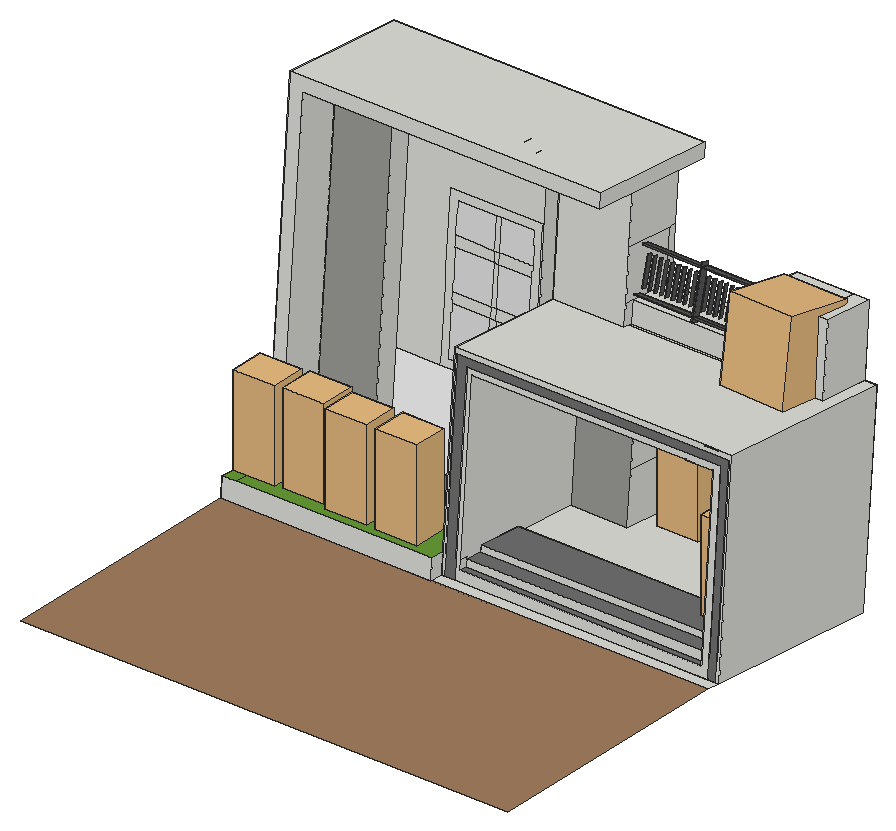
# SketchUp Ruby script. Lengths in inches.
U = 1.inch
M = Sketchup.active_model
def pt(a) = Geom::Point3d.new(a.map { |v| v * U })
def face(e, loops, mat)
  f = e.add_face(loops[0].map { |a| pt(a) })
  loops[1..].each { |l| e.add_face(l.map { |a| pt(a) }).erase! }
  f.material = f.back_material = mat if mat
  f
end
# faces: each face lists its corners as indices into pts; further lists are holes
def faces(e, pts, list, mat = nil) = list.each { |f| face(e, (f[0].is_a?(Array) ? f : [f]).map { |l| l.map { |i| pts[i] } }, mat) }
# xy, xz, yz: faces in a plane at the given z, y or x. An outline is a flat list of corners, or four numbers for a rectangle; further outlines are holes
def ring(l) = l.size == 4 ? [[l[0], l[1]], [l[2], l[1]], [l[2], l[3]], [l[0], l[3]]] : l.each_slice(2).to_a
def flat(e, list, mat, &to3) = list.each { |f| face(e, (f[0].is_a?(Array) ? f : [f]).map { |l| ring(l).map { |u, v| to3.(u, v) } }, mat) }
def xy(e, z, list, mat = nil) = flat(e, list, mat) { |x, y| [x, y, z] }
def xz(e, y, list, mat = nil) = flat(e, list, mat) { |x, z| [x, y, z] }
def yz(e, x, list, mat = nil) = flat(e, list, mat) { |y, z| [x, y, z] }
def lines(e, pts, list) = list.each { |a, b| e.add_line(pt(pts[a]), pt(pts[b])) }
# prism: a flat outline (further loops are holes) pulled along v
def prism(e, loops, v, mat = nil)
  f = face(e, loops, mat); d = Geom::Vector3d.new(v.map { |x| x * U })
  f.pushpull(f.normal.samedirection?(d) ? d.length : -d.length)
end
def box(e, o, s, mat = nil) = prism(e, [[o, [o[0] + s[0], o[1], o[2]], [o[0] + s[0], o[1] + s[1], o[2]], [o[0], o[1] + s[1], o[2]]]], [0, 0, s[2]], mat)
def at(x, y, z, deg = 0) = Geom::Transformation.translation(pt([x, y, z])) * Geom::Transformation.rotation(ORIGIN, Z_AXIS, deg.degrees)
def axes(o, x, y, z) = Geom::Transformation.new([*x, 0, *y, 0, *z, 0, *pt(o).to_a, 1])
def part(name) = M.definitions.add(name)
# library, detail: a bought-in or finely detailed component or shape, given as its bounding box
def library(name, o, s) = part(name).tap { |d| box(d.entities, o, s) }
def detail(e, o, s) = box(e.add_group.entities, o, s)
def put(e, d, t, mat = nil) = e.add_instance(d, t).tap { |i| i.material = mat if mat }
def group(e, t, mat = nil) = e.add_group.tap { |g| g.transformation = t; g.material = mat if mat }.entities
root = M.entities
M.materials.add("M (5)").color = [89, 89, 89]
M.materials.add("M (7)").color = [139, 146, 159]
M.materials.add("[0128_White]").color = [255, 255, 255]
M.materials.add("[Cladding Siding Tan]").color = [162, 126, 95]
M.materials.add("[Color M05]").color = [114, 114, 114]
M.materials.add("[Concrete Block 8x8 Gray]").color = [157, 158, 154]
M.materials.add("[Grass Dark Green]").color = [106, 157, 55]
M.materials.add("[Mirror 02]").color = [229, 229, 229]
c1 = library("Sphere Light",[-0.01,-0.01,-0.01],[0.02,0.02,0.02])
c2 = library("Sphere Light\#2",[-3.2,-3.2,-3.2],[6.4,6.4,6.4])
c3 = library("Sphere Light\#3",[-3.51,-3.51,-3.51],[7.02,7.02,7.02])
c4 = library("Sphere Light\#4",[-3.28,-3.28,-3.28],[6.56,6.56,6.56])
c5 = library("Sphere Light\#6",[-4.5625,-4.5625,-4.5625],[9.125,9.125,9.125])
c6 = library("Sphere Light\#7",[-3.84,-3.84,-3.84],[7.68,7.68,7.68])
c7 = library("Sphere Light\#8",[-4.49,-4.49,-4.49],[8.98,8.98,8.98])
c8 = library("Sphere Light\#9",[-5.16,-5.16,-5.16],[10.32,10.32,10.32])
c9 = library("PINTU+6+YA",[0,-0.6875,0],[35.83,8.07,80.71])
c10 = library("Sphere Light\#10",[-4.25,-4.25,-4.25],[8.5,8.5,8.5])
c11 = library("TS_VASO+GANCHOS-PARA-PENDURAR\#1",[-17.61,-15.74,-70.29],[36.55,50.24,77.96])
c12 = library("Group_2",[-1.28,-0.39,0],[21.22,20.51,48.44])
c13 = library("Sphere Light\#11",[-1.79,-1.79,-1.79],[3.58,3.58,3.58])
c14 = part("Railing post")
box(c14.entities,[0,-0.79,0],[1.18,1.58,46.0625],"M (5)")
c15 = part("Horizontal rails")
box(c15.entities,[0,-0.79,0],[54.52,1.58,1.18],"M (5)")
box(c15.entities,[55.7,-0.79,0],[54.54,1.58,1.18],"M (5)")
xy(c15.entities,38.58,[[55.7,-0.79,58.22,0.79]])
xy(c15.entities,38.58,[[46.34,-0.79,51.99,0.79],[51.99,-0.79,54.52,0.79],[58.22,-0.79,63.67,0.79],[63.67,-0.79,69.12,0.79],[69.12,-0.79,74.57,0.79],
  [74.57,-0.79,80.02,0.79],[80.02,-0.79,85.47,0.79],[85.47,-0.79,90.93,0.79],[90.93,-0.79,96.375,0.79],[96.375,-0.79,101.83,0.79],
  [101.83,-0.79,107.48,0.79],[107.48,-0.79,110.24,0.79]],"M (5)")
xy(c15.entities,38.58,[[0,-0.79,2.73,0.79],[2.73,-0.79,5.45,0.79],[5.45,-0.79,8.18,0.79],[8.18,-0.79,13.63,0.79],[13.63,-0.79,19.08,0.79],
  [19.08,-0.79,24.53,0.79],[24.53,-0.79,29.98,0.79],[29.98,-0.79,35.4375,0.79],[35.4375,-0.79,40.89,0.79],[40.89,-0.79,46.34,0.79]],"M (7)")
xy(c15.entities,39.76,[[0,-0.79,54.52,0.79],[55.7,-0.79,110.24,0.79]],"M (5)")
xz(c15.entities,-0.79,[[0,38.58,54.52,39.76],[55.7,38.58,110.24,39.76]],"M (5)")
xz(c15.entities,0.79,[[0,38.58,54.52,39.76],[55.7,38.58,110.24,39.76]],"M (5)")
yz(c15.entities,0,[[-0.79,38.58,0.79,39.76]],"M (7)")
yz(c15.entities,54.52,[[-0.79,38.58,0.79,39.76]],"M (5)")
yz(c15.entities,55.7,[[-0.79,38.58,0.79,39.76]])
yz(c15.entities,110.24,[[-0.79,38.58,0.79,39.76]],"M (5)")
c16 = part("Railing balusters")
xz(c16.entities,0,[[0,0,0.79,26.38],[5.45,0,6.24,26.38],[10.9,0,11.69,26.38],[16.35,0,17.14,26.38],[21.81,0,22.59,26.38],
  [27.26,0,28.05,26.38],[32.71,0,33.5,26.38],[38.16,0,38.95,26.38],[43.61,0,44.4,26.38],[55.68,0,56.46,26.38],
  [61.13,0,61.91,26.38],[66.58,0,67.37,26.38],[72.03,0,72.82,26.38],[77.48,0,78.27,26.38],[82.93,0,83.72,26.38],
  [88.39,0,89.17,26.38],[93.84,0,94.625,26.38],[99.29,0,100.08,26.38]],"M (5)")
xz(c16.entities,0.79,[[0,0,0.79,26.38],[5.45,0,6.24,26.38],[10.9,0,11.69,26.38],[16.35,0,17.14,26.38],[21.81,0,22.59,26.38],
  [27.26,0,28.05,26.38],[32.71,0,33.5,26.38],[38.16,0,38.95,26.38],[43.61,0,44.4,26.38],[55.68,0,56.46,26.38],
  [61.13,0,61.91,26.38],[66.58,0,67.37,26.38],[72.03,0,72.82,26.38],[77.48,0,78.27,26.38],[82.93,0,83.72,26.38],
  [88.39,0,89.17,26.38],[93.84,0,94.625,26.38],[99.29,0,100.08,26.38]],"M (5)")
yz(c16.entities,0,[[0,0,0.79,26.38]],"M (5)")
yz(c16.entities,0.79,[[0,0,0.79,26.38]],"M (5)")
yz(c16.entities,5.45,[[0,0,0.79,26.38]],"M (5)")
yz(c16.entities,6.24,[[0,0,0.79,26.38]],"M (5)")
yz(c16.entities,10.9,[[0,0,0.79,26.38]],"M (5)")
yz(c16.entities,11.69,[[0,0,0.79,26.38]],"M (5)")
yz(c16.entities,16.35,[[0,0,0.79,26.38]],"M (5)")
yz(c16.entities,17.14,[[0,0,0.79,26.38]],"M (5)")
yz(c16.entities,21.81,[[0,0,0.79,26.38]],"M (5)")
yz(c16.entities,22.59,[[0,0,0.79,26.38]],"M (5)")
yz(c16.entities,27.26,[[0,0,0.79,26.38]],"M (5)")
yz(c16.entities,28.05,[[0,0,0.79,26.38]],"M (5)")
yz(c16.entities,32.71,[[0,0,0.79,26.38]],"M (5)")
yz(c16.entities,33.5,[[0,0,0.79,26.38]],"M (5)")
yz(c16.entities,38.16,[[0,0,0.79,26.38]],"M (5)")
yz(c16.entities,38.95,[[0,0,0.79,26.38]],"M (5)")
yz(c16.entities,43.61,[[0,0,0.79,26.38]],"M (5)")
yz(c16.entities,44.4,[[0,0,0.79,26.38]],"M (5)")
yz(c16.entities,55.68,[[0,0,0.79,26.38]],"M (5)")
yz(c16.entities,56.46,[[0,0,0.79,26.38]],"M (5)")
yz(c16.entities,61.13,[[0,0,0.79,26.38]],"M (5)")
yz(c16.entities,61.91,[[0,0,0.79,26.38]],"M (5)")
yz(c16.entities,66.58,[[0,0,0.79,26.38]],"M (5)")
yz(c16.entities,67.37,[[0,0,0.79,26.38]],"M (5)")
yz(c16.entities,72.03,[[0,0,0.79,26.38]],"M (5)")
yz(c16.entities,72.82,[[0,0,0.79,26.38]],"M (5)")
yz(c16.entities,77.48,[[0,0,0.79,26.38]],"M (5)")
yz(c16.entities,78.27,[[0,0,0.79,26.38]],"M (5)")
yz(c16.entities,82.93,[[0,0,0.79,26.38]],"M (5)")
yz(c16.entities,83.72,[[0,0,0.79,26.38]],"M (5)")
yz(c16.entities,88.39,[[0,0,0.79,26.38]],"M (5)")
yz(c16.entities,89.17,[[0,0,0.79,26.38]],"M (5)")
yz(c16.entities,93.84,[[0,0,0.79,26.38]],"M (5)")
yz(c16.entities,94.625,[[0,0,0.79,26.38]],"M (5)")
yz(c16.entities,99.29,[[0,0,0.79,26.38]],"M (5)")
yz(c16.entities,100.08,[[0,0,0.79,26.38]],"M (5)")
xy(root,21.39,[[0,0,181.29,93.04]],"[Cladding Siding Tan]")
yz(root,0,[[162.59,15.42,98.14,20.95,93.04,21.39,93.66,28.68,114.9,26.86,125.41,149.41,173.73,145.27]])
yz(root,5.0625,[[163.22,22.72,163.32,23.92,130.44,26.74,115,28.07,114.9,26.86],[163.32,23.92,173.3,140.22,140.42,143.04,130.44,26.74],[130.44,26.74,140.42,143.04,124.97,144.37,115,28.07]])
yz(root,26.62,[[138.23,26.08,141.13,59.9,148.2,142.375,140.42,143.04,130.44,26.74]])
yz(root,78.16,[[165.15,15.21,162.59,15.42,163.22,22.72,165.77,22.5],[162.59,15.42,163.22,22.72,98.77,28.25,98.14,20.95],[98.14,20.95,98.77,28.25,93.66,28.68,93.04,21.39],[165.77,22.5,163.22,22.72,163.32,23.92,165.875,23.7],[163.22,22.72,98.77,28.25,98.87,29.45,138.23,26.08,163.32,23.92],
  [165.875,23.7,163.32,23.92,173.3,140.22,175.85,140.01],[163.32,23.92,173.3,140.22,154.24,141.86,149.8125,90.23,143.77,90.75,141.13,59.9,138.23,26.08],[138.23,26.08,98.87,29.45,104.42,94.12,143.77,90.75,141.13,59.9],[149.8125,90.23,154.24,141.86,148.2,142.375,143.77,90.75]])
yz(root,79.13,[[100.82,28.07,106.31,92.02,104.25,92.2,98.77,28.25]])
yz(root,83.04,[[100.82,28.07,98.77,28.25,104.02,89.46,106.07,89.28]])
yz(root,84.88,[[149.77,23.87,154.84,83.05,103.84,87.43,98.77,28.25,101.51,28.01,101.46,27.41,107.76,26.87,107.8125,27.47,107.92,28.67,107.96,29.15,125.35,27.66,125.31,27.18,125.2,25.98],[125.2,25.98,107.8125,27.47,107.92,28.67,125.31,27.18],[125.31,27.18,107.92,28.67,107.96,29.15,125.35,27.66]])
yz(root,104.71,[[153.11,89.94,153.76,97.51,150.46,97.8,149.8125,90.23,152.05,90.04],[172.07,95.94,173.64,114.19,171.08,114.41,169.52,96.16],[169.52,96.16,171.08,114.41,152.03,116.04,150.46,97.8,153.76,97.51],[173.64,114.19,175.85,140.01,173.3,140.22,154.24,141.86,152.03,116.04,171.08,114.41]])
yz(root,105.9375,[[165.77,22.5,167.35,40.95,151.35,42.32,149.77,23.87],[167.35,40.95,169.69,68.23,153.69,69.6,151.35,42.32],[169.69,68.23,170.84,81.57,170.85,81.68,154.84,83.05,153.69,69.6]])
yz(root,115.65,[[173.3,140.22,173.73,145.27,125.41,149.41,124.97,144.37]])
yz(root,150.09,[[172.07,95.94,169.52,96.16,171.08,114.41,173.64,114.19],[169.52,96.16,155.82,97.34,157.38,115.58,171.08,114.41],[155.8,97.18,155.82,97.34,153.76,97.51,153.75,97.35]])
yz(root,164.56,[[170.84,81.57,103.83,87.32,103.84,87.43,170.85,81.68]])
yz(root,171.28,[[171.41,88.27,171.42,88.375,168.87,88.59,168.86,88.48],[153.11,89.94,152.05,90.04,152.69,97.44,153.75,97.35],[155.8,97.18,153.75,97.35,152.69,97.44,154.27,115.85,157.38,115.58],[173.64,114.19,157.38,115.58,154.27,115.85,154.28,115.96,173.64,114.3]])
yz(root,174.57,[[[165.77,22.5,125.2,25.98,125.35,27.66,107.96,29.15,107.8125,27.47,107.76,26.87,101.46,27.41,98.72,27.65,103.83,87.32,170.84,81.57],[161.79,43.81,163.9375,68.91,154.16,69.74,152.01,44.65]],[125.2,25.98,125.35,27.66,107.96,29.15,107.8125,27.47],[161.79,43.81,152.01,44.65,154.16,69.74,163.9375,68.91]])
yz(root,176.84,[[171.41,88.27,168.86,88.48,168.87,88.59,171.42,88.375],[171.42,88.375,173.64,114.3,154.28,115.96,152.05,90.04,168.87,88.59]])
yz(root,177.23,[[100.77,27.47,101.37,34.42,99.3125,34.6,98.72,27.65],[101.37,34.42,106.07,89.28,104.02,89.46,99.3125,34.6]])
yz(root,180.19,[[100.77,27.47,98.72,27.65,104.25,92.2,106.31,92.02]])
yz(root,181.29,[[165.15,15.21,171.42,88.375,104.42,94.12,98.14,20.95]])
p = [[78.16,98.14,20.95],[78.16,162.59,15.42],[78.16,165.15,15.21],[181.29,165.15,15.21],[181.29,98.14,20.95],[180.19,98.14,20.95],
  [177.23,98.14,20.95],[83.04,98.14,20.95],[79.13,98.14,20.95],[78.16,175.85,140.01],[78.16,165.875,23.7],[78.16,165.77,22.5],
  [181.29,171.42,88.375],[176.84,171.42,88.375],[176.84,171.41,88.27],[171.28,171.41,88.27],[171.28,171.42,88.375],[176.84,173.64,114.3],
  [171.28,173.64,114.3],[171.28,173.64,114.19],[150.09,173.64,114.19],[150.09,172.07,95.94],[104.71,172.07,95.94],[104.71,173.64,114.19],
  [104.71,175.85,140.01],[105.9375,169.69,68.23],[105.9375,170.84,81.57],[105.9375,170.85,81.68],[164.56,170.85,81.68],[164.56,170.84,81.57],
  [174.57,170.84,81.57],[174.57,165.77,22.5],[105.9375,165.77,22.5],[105.9375,167.35,40.95],[0,98.14,20.95],[0,162.59,15.42],
  [0,173.73,145.27],[115.65,173.73,145.27],[115.65,173.3,140.22],[104.71,173.3,140.22],[78.16,173.3,140.22],[26.62,173.3,140.22],
  [5.0625,173.3,140.22],[5.0625,163.32,23.92],[5.0625,163.22,22.72],[78.16,163.22,22.72],[0,93.04,21.39],[78.16,93.04,21.39],
  [181.29,93.04,21.39],[180.19,104.25,92.2],[180.19,98.72,27.65],[181.29,104.42,94.12],[176.84,104.42,94.12],[176.84,104.41,94.01],
  [171.28,104.41,94.01],[171.28,104.42,94.12],[78.16,104.42,94.12],[78.16,98.87,29.45],[78.16,98.77,28.25],[79.13,98.77,28.25],
  [79.13,104.25,92.2],[178.75,104.25,92.2],[83.04,98.77,28.25],[83.04,104.02,89.46],[177.23,104.02,89.46],[177.23,99.3125,34.6],
  [177.23,98.72,27.65],[174.57,103.83,87.32],[174.57,98.72,27.65],[174.55,98.44,24.41],[84.86,98.49,25.01],[84.88,98.77,28.25],
  [84.88,103.84,87.43],[164.56,103.84,87.43],[164.56,103.83,87.32],[78.16,93.66,28.68],[5.0625,93.66,28.68],[0,93.66,28.68],
  [84.88,149.77,23.87],[84.88,125.2,25.98],[174.57,125.2,25.98],[105.9375,149.77,23.87],[114.1875,169.69,68.23],[114.1875,167.35,40.95],
  [141.68,169.63,67.53],[156.43,169.63,67.53],[156.43,166.55,31.53],[141.68,166.55,31.53],[134.875,166.79,34.34],[123.6875,166.79,34.34],
  [123.6875,169.63,67.53],[134.875,169.63,67.53],[5.0625,114.9,26.86],[78.16,163.32,23.92],[26.62,163.32,23.92],[26.62,138.23,26.08],
  [26.62,130.44,26.74],[5.0625,130.44,26.74],[78.16,138.23,26.08],[105.9375,151.35,42.32],[105.9375,153.69,69.6],[105.9375,154.84,83.05],
  [84.88,154.84,83.05],[174.55,101.18,24.17],[84.86,101.23,24.77],[174.57,101.46,27.41],[84.88,101.46,27.41],[84.88,101.51,28.01],
  [84.88,125.31,27.18],[84.88,125.35,27.66],[174.57,125.35,27.66],[78.16,141.13,59.9],[77.59,141.13,59.9],[43.28,141.13,59.9],
  [26.62,141.13,59.9],[26.62,140.42,143.04],[5.0625,140.42,143.04],[0,114.9,26.86],[174.57,107.76,26.87],[84.88,107.76,26.87],
  [174.57,107.96,29.15],[84.88,107.96,29.15],[84.88,107.92,28.67],[84.88,107.8125,27.47],[174.57,107.8125,27.47],[0,125.41,149.41],
  [5.0625,115,28.07],[5.0625,124.97,144.37],[115.65,124.97,144.37],[115.65,125.41,149.41],[177.23,100.77,27.47],[180.19,100.77,27.47],
  [180.19,106.31,92.02],[178.75,106.31,92.02],[79.13,106.31,92.02],[79.13,100.82,28.07],[83.04,100.82,28.07],[83.04,106.07,89.28],
  [177.23,106.07,89.28],[177.23,101.37,34.42],[77.59,145.99,116.63],[78.16,143.77,90.75],[78.16,148.2,142.375],[26.62,148.2,142.375],
  [43.28,145.99,116.63],[46.13,144.77,102.43],[46.13,145.75,113.8],[60.4375,145.75,113.8],[62.53,145.75,113.8],[74.75,145.75,113.8],
  [74.75,144.77,102.43],[74.75,144.45,98.6],[74.75,143.22,84.31],[74.75,142.91,80.67],[74.75,141.37,62.74],[62.53,141.37,62.74],
  [60.4375,141.37,62.74],[46.13,141.37,62.74],[46.13,142.91,80.67],[46.13,143.22,84.31],[46.13,144.45,98.6],[60.4375,142.91,80.67],
  [62.53,142.91,80.67],[60.4375,143.22,84.31],[62.53,143.22,84.31],[100.26,122.5,85.83],[99.72,121.2,85.9375],[99.54,119.82,86.06],
  [99.72,118.43,86.17],[100.26,117.14,86.29],[101.11,116.03,86.38],[102.23,115.18,86.45],[103.52,114.65,86.5],[104.91,114.46,86.52],
  [106.31,114.65,86.5],[107.6,115.18,86.45],[108.71,116.03,86.38],[109.57,117.14,86.29],[110.11,118.43,86.17],[110.29,119.82,86.06],
  [110.11,121.2,85.9375],[109.57,122.5,85.83],[108.71,123.6,85.73],[107.6,124.46,85.66],[106.31,124.99,85.61],[104.91,125.17,85.6],
  [103.52,124.99,85.61],[102.23,124.46,85.66],[101.11,123.6,85.73],[127.39,115.75,86.4],[128.34,116.71,86.32],[129,117.89,86.22],
  [129.34,119.2,86.11],[129.33,120.54,85.99],[128.96,121.84,85.88],[128.27,123.01,85.78],[127.31,123.95,85.7],[126.13,124.61,85.64],
  [124.82,124.95,85.62],[123.46,124.94,85.62],[122.16,124.57,85.65],[120.99,123.89,85.71],[120.04,122.92,85.79],[119.38,121.75,85.89],
  [119.04,120.44,86],[119.05,119.09,86.12],[119.42,117.79,86.23],[120.11,116.63,86.33],[121.07,115.6875,86.41],[122.25,115.02,86.47],
  [123.57,114.6875,86.5],[124.92,114.7,86.49],[126.22,115.0625,86.46],[158.82,115.88,86.39],[159.76,116.6,86.33],[160.49,117.55,86.25],
  [160.94,118.64,86.16],[161.1,119.82,86.06],[160.94,120.99,85.96],[160.49,122.09,85.86],[159.76,123.03,85.78],[158.82,123.75,85.72],
  [157.72,124.21,85.68],[156.54,124.36,85.67],[155.36,124.21,85.68],[154.26,123.75,85.72],[153.31,123.03,85.78],[152.59,122.09,85.86],
  [152.13,120.99,85.96],[151.97,119.82,86.06],[152.13,118.64,86.16],[152.59,117.55,86.25],[153.31,116.6,86.33],[154.26,115.88,86.39],
  [155.36,115.43,86.43],[156.54,115.27,86.45],[157.72,115.43,86.43],[142.28,115.94,86.39],[143.21,116.65,86.33],[143.93,117.58,86.25],
  [144.38,118.66,86.16],[144.53,119.82,86.06],[144.38,120.98,85.96],[143.93,122.06,85.86],[143.21,122.99,85.78],[142.28,123.7,85.72],
  [141.2,124.15,85.68],[140.03,124.3,85.67],[138.87,124.15,85.68],[137.78,123.7,85.72],[136.85,122.99,85.78],[136.13,122.06,85.86],
  [135.68,120.98,85.96],[135.53,119.82,86.06],[135.68,118.66,86.16],[136.13,117.58,86.25],[136.85,116.65,86.33],[137.78,115.94,86.39],
  [138.87,115.49,86.43],[140.03,115.33,86.44],[141.2,115.49,86.43],[60.4375,144.45,98.6],[62.53,144.45,98.6],[122.16,124.68,86.89],
  [120.99,123.99,86.95],[127.31,124.06,86.95],[126.13,124.72,86.89],[103.52,125.08,86.67],[102.23,124.55,86.72],[107.6,124.55,86.72],
  [106.31,125.08,86.67],[123.46,125.04,86.86],[124.82,125.06,86.86],[104.91,125.26,86.66],[101.11,123.7,86.79],[100.26,122.59,86.89],
  [109.57,122.59,86.89],[108.71,123.7,86.79],[120.04,123.03,87.04],[128.27,123.11,87.03],[137.78,123.78,86.66],[136.85,123.07,86.72],
  [143.21,123.07,86.72],[142.28,123.78,86.66],[154.26,123.89,87.28],[153.31,123.17,87.34],[159.76,123.17,87.34],[158.82,123.89,87.28],
  [138.87,124.23,86.62],[141.2,124.23,86.62],[155.36,124.34,87.24],[157.72,124.34,87.24],[140.03,124.38,86.61],[156.54,124.5,87.22],
  [99.72,121.3,87],[110.11,121.3,87],[119.38,121.85,87.14],[128.96,121.95,87.13],[136.13,122.14,86.8],[143.93,122.14,86.8],
  [152.59,122.22,87.42],[160.49,122.22,87.42],[99.54,119.91,87.11],[110.29,119.91,87.11],[119.04,120.55,87.25],[129.33,120.65,87.24],
  [135.68,121.06,86.89],[144.38,121.06,86.89],[152.13,121.13,87.51],[160.94,121.13,87.51],[119.05,119.2,87.36],[129.34,119.3,87.35],
  [135.53,119.9,86.99],[144.53,119.9,86.99],[151.97,119.95,87.61],[161.1,119.95,87.61],[119.42,117.9,87.48],[129,118,87.47],
  [99.72,118.52,87.23],[110.11,118.52,87.23],[152.13,118.78,87.71],[160.94,118.78,87.71],[135.68,118.74,87.09],[144.38,118.74,87.09],
  [120.11,116.74,87.57],[136.13,117.66,87.18],[136.85,116.73,87.26],[143.21,116.73,87.26],[143.93,117.66,87.18],[128.34,116.82,87.57],
  [100.26,117.23,87.34],[109.57,117.23,87.34],[152.59,117.68,87.81],[160.49,117.68,87.81],[121.07,115.79,87.66],[127.39,115.86,87.65],
  [137.78,116.02,87.32],[142.28,116.02,87.32],[153.31,116.74,87.89],[154.26,116.01,87.95],[158.82,116.01,87.95],[159.76,116.74,87.89],
  [101.11,116.12,87.4375],[108.71,116.12,87.4375],[122.25,115.13,87.71],[126.22,115.17,87.71],[102.23,115.27,87.51],[107.6,115.27,87.51],
  [138.87,115.57,87.36],[140.03,115.41,87.375],[141.2,115.57,87.36],[155.36,115.5625,87.99],[156.54,115.41,88],[157.72,115.5625,87.99],
  [103.52,114.74,87.56],[104.91,114.55,87.57],[106.31,114.74,87.56],[123.57,114.79,87.74],[124.92,114.81,87.74],[171.28,168.86,88.48],
  [176.84,168.86,88.48],[176.84,168.87,88.59],[176.84,152.05,90.04],[171.28,152.05,90.04],[104.71,152.05,90.04],[104.71,149.8125,90.23],
  [78.16,149.8125,90.23],[171.28,168.87,88.59],[171.28,153.11,89.94],[104.71,153.11,89.94],[150.09,153.75,97.35],[150.09,153.76,97.51],
  [104.71,153.76,97.51],[171.28,153.75,97.35],[78.16,152.05,90.04],[171.28,154.28,115.96],[171.28,154.27,115.85],[171.28,152.69,97.44],
  [176.84,154.28,115.96],[104.71,150.46,97.8],[104.71,152.03,116.04],[104.71,154.24,141.86],[78.16,154.24,141.86],[104.71,169.52,96.16],
  [150.09,169.52,96.16],[150.09,155.82,97.34],[171.28,155.8,97.18],[150.09,155.8,97.18],[171.28,157.38,115.58],[150.09,157.38,115.58],
  [60.4375,144.77,102.43],[62.53,144.77,102.43],[150.09,171.08,114.41],[108.11,152.15,142.04],[107.08,152.58,142],[105.98,152.72,141.99],
  [104.88,152.58,142],[103.86,152.15,142.04],[102.98,151.48,142.1],[102.3,150.6,142.17],[101.88,149.58,142.26],[101.73,148.49,142.35],
  [101.88,147.39,142.45],[102.3,146.37,142.53],[102.98,145.49,142.61],[103.86,144.82,142.67],[104.88,144.4,142.7],[105.98,144.25,142.72],
  [107.08,144.4,142.7],[108.11,144.82,142.67],[108.99,145.49,142.61],[109.67,146.37,142.53],[110.09,147.39,142.45],[110.23,148.49,142.35],
  [110.09,149.58,142.26],[109.67,150.6,142.17],[108.99,151.48,142.1],[107.52,136.93,143.34],[107.17,137.78,143.27],[106.61,138.5,143.21],
  [105.89,139.05,143.16],[105.04,139.4,143.13],[104.14,139.52,143.12],[103.23,139.4,143.13],[102.39,139.05,143.16],[101.66,138.5,143.21],
  [101.1,137.78,143.27],[100.75,136.93,143.34],[100.64,136.03,143.42],[100.75,135.13,143.5],[101.1,134.29,143.57],[101.66,133.57,143.63],
  [102.39,133.01,143.68],[103.23,132.66,143.71],[104.14,132.54,143.72],[105.04,132.66,143.71],[105.89,133.01,143.68],[106.61,133.57,143.63],
  [107.17,134.29,143.57],[107.52,135.13,143.5],[107.64,136.03,143.42],[84.72,136.93,143.34],[84.37,137.78,143.27],[83.82,138.5,143.21],
  [83.09,139.05,143.16],[82.25,139.4,143.13],[81.34,139.52,143.12],[80.44,139.4,143.13],[79.59,139.05,143.16],[78.87,138.5,143.21],
  [78.31,137.78,143.27],[77.96,136.93,143.34],[77.84,136.03,143.42],[77.96,135.13,143.5],[78.31,134.29,143.57],[78.87,133.57,143.63],
  [79.59,133.01,143.68],[80.44,132.66,143.71],[81.34,132.54,143.72],[82.25,132.66,143.71],[83.09,133.01,143.68],[83.82,133.57,143.63],
  [84.37,134.29,143.57],[84.72,135.13,143.5],[84.84,136.03,143.42],[58.86,138.1875,143.24],[58.37,137.56,143.29],[58.0625,136.82,143.35],
  [57.96,136.03,143.42],[58.0625,135.24,143.49],[58.37,134.51,143.55],[58.86,133.875,143.61],[59.49,133.39,143.65],[60.23,133.08,143.67],
  [61.02,132.98,143.68],[61.82,133.08,143.67],[62.55,133.39,143.65],[63.1875,133.875,143.61],[63.67,134.51,143.55],[63.98,135.24,143.49],
  [64.09,136.03,143.42],[63.98,136.82,143.35],[63.67,137.56,143.29],[63.1875,138.1875,143.24],[62.55,138.67,143.19],[61.82,138.98,143.17],
  [61.02,139.08,143.16],[60.23,138.98,143.17],[59.49,138.67,143.19],[42.09,134.51,143.55],[42.39,135.24,143.49],[42.5,136.03,143.42],
  [42.39,136.82,143.35],[42.09,137.56,143.29],[41.6,138.1875,143.24],[40.97,138.67,143.19],[40.23,138.98,143.17],[39.43,139.08,143.16],
  [38.64,138.98,143.17],[37.9,138.67,143.19],[37.27,138.1875,143.24],[36.78,137.56,143.29],[36.48,136.82,143.35],[36.37,136.03,143.42],
  [36.48,135.24,143.49],[36.78,134.51,143.55],[37.27,133.875,143.61],[37.9,133.39,143.65],[38.64,133.08,143.67],[39.43,132.98,143.68],
  [40.23,133.08,143.67],[40.97,133.39,143.65],[41.6,133.875,143.61],[103.86,152.26,143.22],[102.98,151.58,143.28],[108.99,151.58,143.28],
  [108.11,152.26,143.22],[104.88,152.68,143.18],[107.08,152.68,143.18],[105.98,152.82,143.17],[102.3,150.71,143.35],[109.67,150.71,143.35],
  [101.88,149.69,143.44],[110.09,149.69,143.44],[101.73,148.59,143.54],[110.23,148.59,143.54],[101.88,147.49,143.63],[102.3,146.47,143.72],
  [109.67,146.47,143.72],[110.09,147.49,143.63],[102.98,145.59,143.79],[108.99,145.59,143.79],[103.86,144.92,143.85],[108.11,144.92,143.85],
  [104.88,144.5,143.89],[105.98,144.35,143.9],[107.08,144.5,143.89],[80.44,139.5,144.31],[79.59,139.15,144.34],[83.09,139.15,144.34],
  [82.25,139.5,144.31],[103.23,139.56,145],[102.39,139.21,145.03],[105.89,139.21,145.03],[105.04,139.56,145],[81.34,139.62,144.3],
  [104.14,139.68,144.99],[37.27,138.29,144.42],[36.78,137.66,144.47],[42.09,137.66,144.47],[41.6,138.29,144.42],[58.86,138.34,144.98],
  [58.37,137.71,145.03],[63.67,137.71,145.03],[63.1875,138.34,144.98],[78.87,138.6,144.39],[78.31,137.875,144.45],[84.37,137.875,144.45],
  [83.82,138.6,144.39],[101.66,138.66,145.08],[101.1,137.94,145.14],[107.17,137.94,145.14],[106.61,138.66,145.08],[37.9,138.78,144.375],
  [40.97,138.78,144.375],[59.49,138.82,144.9375],[62.55,138.82,144.9375],[38.64,139.08,144.35],[40.23,139.08,144.35],[60.23,139.13,144.91],
  [61.82,139.13,144.91],[39.43,139.18,144.34],[61.02,139.23,144.9],[77.96,137.04,144.53],[77.84,136.13,144.6],[84.84,136.13,144.6],
  [84.72,137.04,144.53],[100.75,137.09,145.21],[100.64,136.19,145.29],[107.64,136.19,145.29],[107.52,137.09,145.21],[36.48,136.92,144.54],
  [42.39,136.92,144.54],[58.0625,136.97,145.1],[63.98,136.97,145.1],[77.96,135.23,144.68],[84.72,135.23,144.68],[100.75,135.29,145.37],
  [107.52,135.29,145.37],[36.37,136.13,144.6],[36.48,135.34,144.67],[42.39,135.34,144.67],[42.5,136.13,144.6],[57.96,136.18,145.16],
  [58.0625,135.39,145.23],[63.98,135.39,145.23],[64.09,136.18,145.16],[78.31,134.39,144.75],[84.37,134.39,144.75],[101.1,134.45,145.4375],
  [107.17,134.45,145.4375],[36.78,134.61,144.73],[42.09,134.61,144.73],[58.37,134.66,145.29],[63.67,134.66,145.29],[78.87,133.67,144.81],
  [79.59,133.11,144.86],[83.09,133.11,144.86],[83.82,133.67,144.81],[101.66,133.73,145.5],[102.39,133.17,145.55],[105.89,133.17,145.55],
  [106.61,133.73,145.5],[37.9,133.49,144.83],[38.64,133.1875,144.86],[40.23,133.1875,144.86],[40.97,133.49,144.83],[59.49,133.54,145.39],
  [60.23,133.23,145.42],[61.82,133.23,145.42],[62.55,133.54,145.39],[37.27,133.98,144.79],[41.6,133.98,144.79],[58.86,134.02,145.35],
  [63.1875,134.02,145.35],[80.44,132.76,144.89],[81.34,132.65,144.9],[82.25,132.76,144.89],[103.23,132.82,145.58],[104.14,132.7,145.59],
  [105.04,132.82,145.58],[39.43,133.08,144.87],[61.02,133.13,145.43],[-623.75,678.73,0],[-623.75,-254.02,0],[-107.6875,-254.02,0]]
faces(root,p,[[0,1,2,3,4,5,6,7,8],[[9,10,11,2,3,12,13,14,15,16,13,17,18,19,20,21,22,23,24],[25,26,27,28,29,30,31,32,33]],[1,0,34,35],[35,36,37,38,39,40,41,42,43,44,45,1],[46,34,0,47],[5,4,48,47,0,8,7,6],[49,50,5,4,51,52,53,54,55,56,57,58,0,8,59,60,61],[[7,6,66,65,64,63,62],[67,68,69,70,71,72,73,74]],
  [75,76,77,46,47],[78,79,80,31,32,81],[[30,29,26,25,82,83,33,32,31],[84,85,86,87],[88,89,90,91]],[44,45,93,94,43],[43,94,95,96,97],[94,93,98,95],[43,42,41,40,93,94],[68,105,103,69],
  [103,105,106,107,104],[107,71,70,104],[80,79,108,109,110],[120,121,122,123,119,118,124],[125,117,92,126,127,128,129],[130,131,132,133,134,135,136,137,138,139],[85,84,87,86],[89,88,91,90],
  [25,33,83,82],[140,112,111,141,142,143,114,113,144],[[140,144,113,112],[145,146,147,148,149,150,151,152,153,154,155,156,157,158,159,160]],[155,162,161,156],[161,163,159,158],[162,164,163,161],[164,162,153,152],[74,29,30,67],
  [27,26,29,28],[[102,101,27,28,73,72],[165,166,167,168,169,170,171,172,173,174,175,176,177,178,179,180,181,182,183,184,185,186,187,188],[189,190,191,192,193,194,195,196,197,198,199,200,201,202,203,204,205,206,207,208,209,210,211,212],[213,214,215,216,217,218,219,220,221,222,223,224,225,226,227,228,229,230,231,232,233,234,235,236],[237,238,239,240,241,242,243,244,245,246,247,248,249,250,251,252,253,254,255,256,257,258,259,260]],[261,163,164,262],[201,200,263,264],[197,196,265,266],[187,186,267,268],[184,183,269,270],[200,199,271,263],
  [198,197,266,272],[199,198,272,271],[186,185,273,267],[185,184,270,273],[165,188,274,275],[182,181,276,277],[202,201,264,278],[196,195,279,265],
  [250,249,280,281],[245,244,282,283],[226,225,284,285],[221,220,286,287],[188,187,268,274],[183,182,277,269],[249,248,288,280],[246,245,283,289],
  [225,224,290,284],[222,221,287,291],[248,247,292,288],[247,246,289,292],[224,223,293,290],[223,222,291,293],[166,165,275,294],[181,180,295,276],
  [203,202,278,296],[195,194,297,279],[251,250,281,298],[244,243,299,282],[227,226,285,300],[220,219,301,286],[167,166,294,302],[180,179,303,295],
  [204,203,296,304],[194,193,305,297],[252,251,298,306],[243,242,307,299],[228,227,300,308],[219,218,309,301],[205,204,304,310],[193,192,311,305],
  [253,252,306,312],[242,241,313,307],[229,228,308,314],[218,217,315,309],[206,205,310,316],[192,191,317,311],[168,167,302,318],[179,178,319,303],
  [230,229,314,320],[217,216,321,315],[254,253,312,322],[241,240,323,313],[207,206,316,324],[256,255,325,326],[239,238,327,328],[191,190,329,317],
  [169,168,318,330],[178,177,331,319],[231,230,320,332],[216,215,333,321],[255,254,322,325],[240,239,328,323],[208,207,324,334],[190,189,335,329],
  [257,256,326,336],[238,237,337,327],[233,232,338,339],[214,213,340,341],[170,169,330,342],[177,176,343,331],[232,231,332,338],[215,214,341,333],
  [209,208,334,344],[189,212,345,335],[171,170,342,346],[176,175,347,343],[259,258,348,349],[260,259,349,350],[235,234,351,352],[236,235,352,353],
  [234,233,339,351],[213,236,353,340],[258,257,336,348],[237,260,350,337],[173,172,354,355],[174,173,355,356],[172,171,346,354],[175,174,356,347],
  [210,209,344,357],[211,210,357,358],[212,211,358,345],[327,337,350,349,348,336,326,325,322,312,306,298,281,280,288,292,289,283,282,299,307,313,323,328],[294,275,274,268,267,273,270,269,277,276,295,303,319,331,343,347,356,355,354,346,342,330,318,302],[329,335,345,358,357,344,334,324,316,310,304,296,278,264,263,271,272,266,265,279,297,305,311,317],[341,340,353,352,351,339,338,332,320,314,308,300,285,284,290,293,291,287,286,301,309,315,321,333],[359,360,14,15],
  [361,362,363,364,365,366,141,56,55,52,51,12,13],[361,367,16,13],[360,361,367,359],[367,361,362,363,368],[137,63,64,138],[364,363,368,369],[370,371,372,369,368,373],[364,374,366,365],
  [375,376,377,363,362,378],[366,365,379,380,381,382],[61,60,134,133],[49,61,133,132],[52,55,54,53],[383,384,21,22],[384,383,372,371,385],[373,386,387,370],
  [145,160,261,390],[262,391,390,261],[391,262,151,150],[147,390,391,148],[388,19,20,392,389],[378,17,18,375],[40,39,24,9],[[116,115,143,142,382,381,39,38,128,127],[393,394,395,396,397,398,399,400,401,402,403,404,405,406,407,408,409,410,411,412,413,414,415,416],[417,418,419,420,421,422,423,424,425,426,427,428,429,430,431,432,433,434,435,436,437,438,439,440],[441,442,443,444,445,446,447,448,449,450,451,452,453,454,455,456,457,458,459,460,461,462,463,464],[465,466,467,468,469,470,471,472,473,474,475,476,477,478,479,480,481,482,483,484,485,486,487,488],[489,490,491,492,493,494,495,496,497,498,499,500,501,502,503,504,505,506,507,508,509,510,511,512]],
  [42,41,143,115,116],[41,40,382,142,143],[40,39,381,382],[398,397,513,514],[393,416,515,516],[397,396,517,513],[394,393,516,518],[396,395,519,517],
  [395,394,518,519],[399,398,514,520],[416,415,521,515],[400,399,520,522],[415,414,523,521],[401,400,522,524],[414,413,525,523],[403,402,526,527],
  [412,411,528,529],[402,401,524,526],[413,412,529,525],[404,403,527,530],[411,410,531,528],[405,404,530,532],[410,409,533,531],[407,406,534,535],
  [408,407,535,536],[406,405,532,534],[409,408,536,533],[448,447,537,538],[445,444,539,540],[424,423,541,542],[421,420,543,544],[447,446,545,537],
  [446,445,540,545],[423,422,546,541],[422,421,544,546],[501,500,547,548],[494,493,549,550],[466,465,551,552],[483,482,553,554],[450,449,555,556],
  [443,442,557,558],[426,425,559,560],[419,418,561,562],[500,499,563,547],[495,494,550,564],[465,488,565,551],[484,483,554,566],[449,448,538,555],
  [444,443,558,539],[425,424,542,559],[420,419,562,543],[499,498,567,563],[496,495,564,568],[488,487,569,565],[485,484,566,570],[498,497,571,567],
  [497,496,568,571],[487,486,572,569],[486,485,570,572],[518,516,515,521,523,525,529,528,531,533,536,535,534,532,530,527,526,524,522,520,514,513,517,519],[452,451,573,574],[441,464,575,576],[428,427,577,578],[417,440,579,580],
  [502,501,548,581],[493,492,582,549],[467,466,552,583],[482,481,584,553],[451,450,556,573],[442,441,576,557],[427,426,560,577],[418,417,580,561],
  [453,452,574,585],[464,463,586,575],[429,428,578,587],[440,439,588,579],[504,503,589,590],[491,490,591,592],[469,468,593,594],[480,479,595,596],
  [503,502,581,589],[492,491,592,582],[468,467,583,593],[481,480,596,584],[454,453,585,597],[463,462,598,586],[430,429,587,599],[439,438,600,588],
  [505,504,590,601],[490,489,602,591],[470,469,594,603],[479,478,604,595],[456,455,605,606],[461,460,607,608],[432,431,609,610],[437,436,611,612],
  [508,507,613,614],[511,510,615,616],[473,472,617,618],[476,475,619,620],[507,506,621,613],[512,511,616,622],[472,471,623,617],[477,476,620,624],
  [455,454,597,605],[462,461,608,598],[431,430,599,609],[438,437,612,600],[506,505,601,621],[489,512,622,602],[471,470,603,623],[478,477,624,604],
  [458,457,625,626],[459,458,626,627],[434,433,628,629],[435,434,629,630],[457,456,606,625],[460,459,627,607],[433,432,610,628],[436,435,630,611],
  [509,508,614,631],[510,509,631,615],[474,473,618,632],[475,474,632,619],[557,576,575,586,598,608,607,627,626,625,606,605,597,585,574,573,556,555,538,537,545,540,539,558],[591,602,622,616,615,631,614,613,621,601,590,589,581,548,547,563,567,571,568,564,550,549,582,592],[552,551,565,569,572,570,566,554,553,584,596,595,604,624,620,619,632,618,617,623,603,594,593,583],[561,580,579,588,600,612,611,630,629,628,610,609,599,587,578,577,560,559,542,541,546,544,543,562],
  [37,36,125,129]])
faces(root,p,[[5,50,49,61,60,59,8,7,62,63,64,65,66,6],[103,104,70,69],[105,118,119,106],[109,121,120,110]],"[Color M05]")
faces(root,p,[[45,44,92,76,75,58],[92,117,77,76]],"[Grass Dark Green]")
faces(root,p,[[78,81,99,100,101,102],[97,96,115,116],[388,389,385,387,386]],"[Concrete Block 8x8 Gray]")
faces(root,p,[[98,111,112,113,114,95]],"[0128_White]")
faces(root,p,[[156,161,158,157],[154,153,162,155],[160,159,163,261],[262,164,152,151],[146,145,390,147],[148,391,150,149]],"[Mirror 02]")
lines(root,p,[[633,634],[634,635]])
put(root,c1,axes([39.43,136.03,143.42],[1,0,0],[0,0.08544,0.99634],[0,-0.99634,0.08544]))
put(root,c2,axes([60.73,136.13,144.6],[1,0,0],[0,0.08544,0.99634],[0,-0.99634,0.08544]))
put(root,c3,axes([81.625,136.13,144.6],[1,0,0],[0,0.08544,0.99634],[0,-0.99634,0.08544]))
put(root,c4,axes([39.43,136.03,143.42],[1,0,0],[0,0.08544,0.99634],[0,-0.99634,0.08544]))
put(root,c5,axes([156.54,119.82,86.06],[1,0,0],[0,0.08544,0.99634],[0,-0.99634,0.08544]))
put(root,c6,axes([140.0625,120.71,86.92],[1,0,0],[0,0.08544,0.99634],[0,-0.99634,0.08544]))
put(root,c7,axes([123.65,121.24,87.1875],[1,0,0],[0,0.08544,0.99634],[0,-0.99634,0.08544]))
put(root,c8,axes([104.84,120.3,87.08],[1,0,0],[0,0.08544,0.99634],[0,-0.99634,0.08544]))
put(root,c9,axes([141.68,166.55,31.53],[0.48,0,0],[0,-0.14947,0],[0,0,0.468]))
put(root,c10,axes([105.98,148.49,144.23],[1,0,0],[0,1,0],[0,0,0.55804]))
put(root,c11,axes([165.75,154.29,114.99],[0.03495,0.65043,-0.11124],[-0.48308,0.02415,-0.01055],[-0.00578,0.07489,0.43608]))
put(root,c12,axes([155.79,151.38,23.73],[0.73,0,0],[0,0.62,0],[0,0,0.69]))
put(root,c12,axes([112.02,157.15,23.26],[0.73,0,0],[0,0.62,0],[0,0,0.69]))
put(root,c12,axes([0.93,99.1,28.24],[0.73,0,0],[0,0.62,0],[0,0,0.69]))
put(root,c12,axes([18.68,99.91,28.15],[0.73,0,0],[0,0.62,0],[0,0,0.69]))
put(root,c12,axes([36.46,97.47,28.38],[0.73,0,0],[0,0.62,0],[0,0,0.69]))
put(root,c12,axes([161.02,116.35,28.43],[0.73,0,0],[0,0.62,0],[0,0,0.69]))
put(root,c12,axes([55.4,97.23,28.38],[0.73,0,0],[0,0.62,0],[0,0,0.69]))
put(root,c13,at(103.44,138.51,145.09))
g1 = group(root,at(106.85,153.83,98.85))
put(g1,c14,axes([21.61,-1.25,0.34],[0.39644,0,0],[0,-1.5873,0.42832],[0,0.10551,0.39101]))
put(g1,c15,axes([0,-0.92,1.57],[0.39644,0,0],[0,-1.5873,0.42832],[0,0.10551,0.39101]))
put(g1,c16,axes([2.01,0.41,4.02],[0.39644,0,0],[0,-1.5873,0.42832],[0,0.10551,0.39101]))
